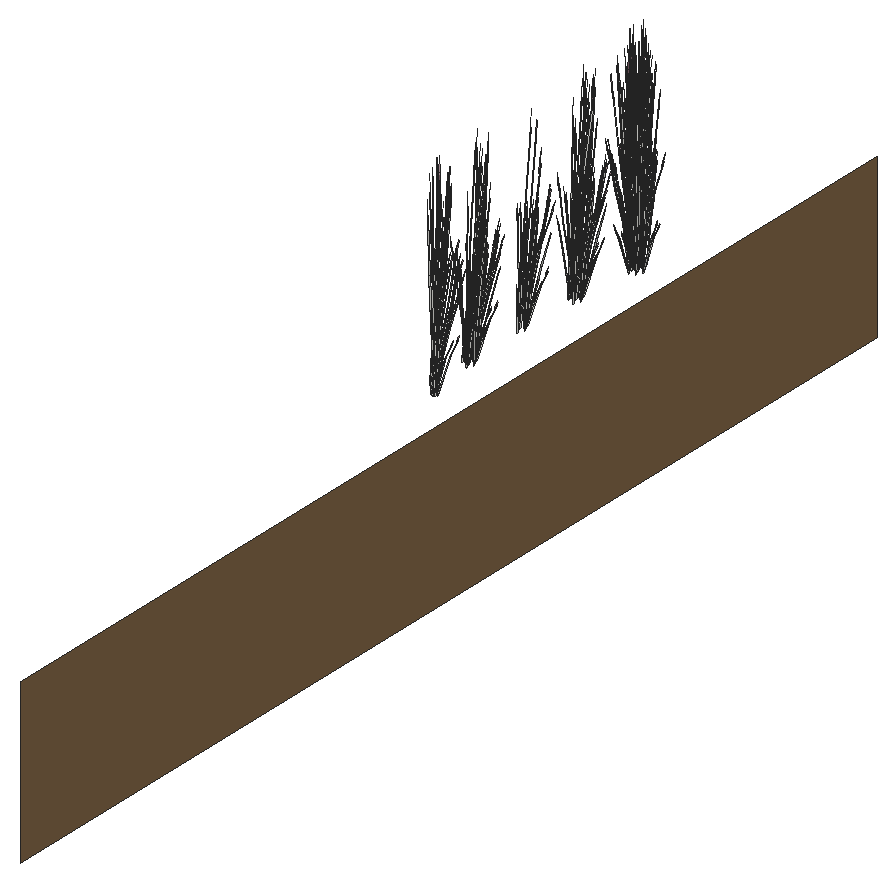
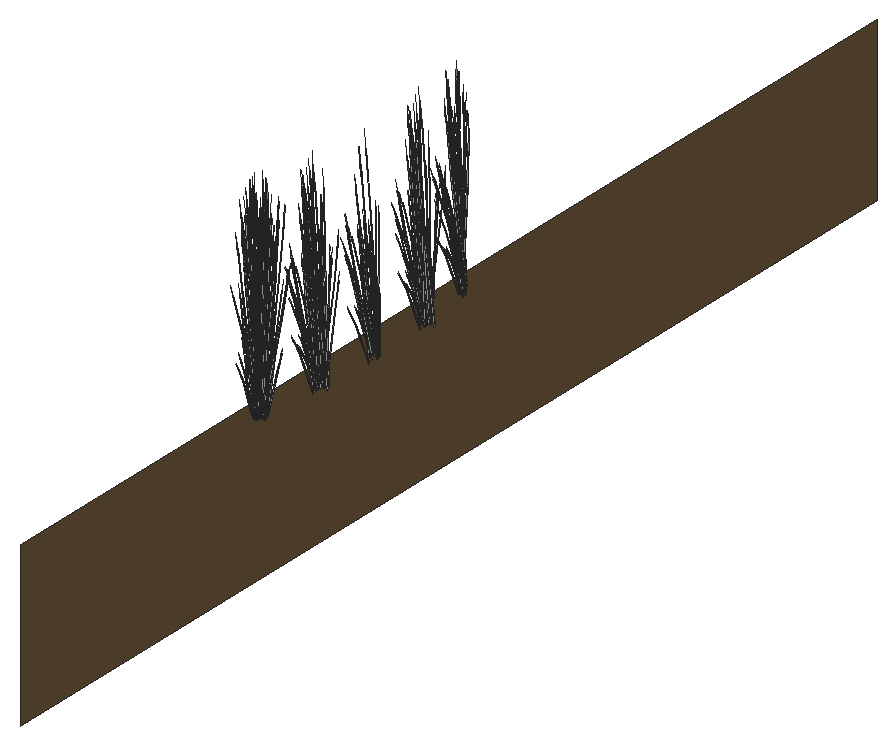
# SketchUp Ruby script. Lengths in inches.
U = 1.inch
M = Sketchup.active_model
def pt(a) = Geom::Point3d.new(a.map { |v| v * U })
def face(e, loops, mat)
  f = e.add_face(loops[0].map { |a| pt(a) })
  loops[1..].each { |l| e.add_face(l.map { |a| pt(a) }).erase! }
  f.material = f.back_material = mat if mat
  f
end
# faces: each face lists its corners as indices into pts; further lists are holes
def faces(e, pts, list, mat = nil) = list.each { |f| face(e, (f[0].is_a?(Array) ? f : [f]).map { |l| l.map { |i| pts[i] } }, mat) }
# xy, xz, yz: faces in a plane at the given z, y or x. An outline is a flat list of corners, or four numbers for a rectangle; further outlines are holes
def ring(l) = l.size == 4 ? [[l[0], l[1]], [l[2], l[1]], [l[2], l[3]], [l[0], l[3]]] : l.each_slice(2).to_a
def flat(e, list, mat, &to3) = list.each { |f| face(e, (f[0].is_a?(Array) ? f : [f]).map { |l| ring(l).map { |u, v| to3.(u, v) } }, mat) }
def xy(e, z, list, mat = nil) = flat(e, list, mat) { |x, y| [x, y, z] }
def xz(e, y, list, mat = nil) = flat(e, list, mat) { |x, z| [x, y, z] }
def yz(e, x, list, mat = nil) = flat(e, list, mat) { |y, z| [x, y, z] }
def lines(e, pts, list) = list.each { |a, b| e.add_line(pt(pts[a]), pt(pts[b])) }
# prism: a flat outline (further loops are holes) pulled along v
def prism(e, loops, v, mat = nil)
  f = face(e, loops, mat); d = Geom::Vector3d.new(v.map { |x| x * U })
  f.pushpull(f.normal.samedirection?(d) ? d.length : -d.length)
end
def box(e, o, s, mat = nil) = prism(e, [[o, [o[0] + s[0], o[1], o[2]], [o[0] + s[0], o[1] + s[1], o[2]], [o[0], o[1] + s[1], o[2]]]], [0, 0, s[2]], mat)
def at(x, y, z, deg = 0) = Geom::Transformation.translation(pt([x, y, z])) * Geom::Transformation.rotation(ORIGIN, Z_AXIS, deg.degrees)
def axes(o, x, y, z) = Geom::Transformation.new([*x, 0, *y, 0, *z, 0, *pt(o).to_a, 1])
def part(name) = M.definitions.add(name)
# library, detail: a bought-in or finely detailed component or shape, given as its bounding box
def library(name, o, s) = part(name).tap { |d| box(d.entities, o, s) }
def detail(e, o, s) = box(e.add_group.entities, o, s)
def put(e, d, t, mat = nil) = e.add_instance(d, t).tap { |i| i.material = mat if mat }
def group(e, t, mat = nil) = e.add_group.tap { |g| g.transformation = t; g.material = mat if mat }.entities
root = M.entities
M.materials.add("LightPink_Translucent").color = [144, 107, 117]
M.materials["LightPink_Translucent"].alpha = 0.75
M.materials.add("Soil_03_1K").color = [122, 96, 67]
c1 = part("blade")
p = [[2.15,0.21,22],[0,0.17,0],[0.09,0.45,0],[2.18,0.31,22],[2.29,0.31,22],[0.38,0.45,0],
  [2.48,0.24,33],[2.49,0.24,33],[2.48,0.22,33]]
faces(c1.entities,p,[[0,1,2,3],[4,5,2,3],[6,3,4,7],[8,0,3,6]])
c2 = part("seeds")
p = [[0.3,-0.1,1.38],[-0.01,-0.03,1.59],[-0.01,-0.03,0.03],[0.14,-0.07,-0.07],[0.29,-0.03,3],[0.15,0.01,3.11]]
faces(c2.entities,p,[[0,1,2,3],[1,0,4,5]],"LightPink_Translucent")
c3 = part("blade with seeds")
put(c3.entities,c1,at(0,0,0))
put(c3.entities,c2,axes([2.4,0.25,30.99],[1.5799,-0.05474,1.17369],[-0.12525,1.92788,0.29478],[-0.07173,-0.02425,1.56792]))
yz(root,410.57,[[0,-48,316.3,0]],"Soil_03_1K")
put(root,c3,axes([402.34,162.62,2.29],[0.15345,0.53576,-0.06012],[-0.43845,0.18773,0],[0.00536,0.01871,1.72173]))
put(root,c3,axes([402.51,163.2,2.03],[-0.32928,-0.11539,-0.30978],[0.08291,-0.40636,0.30978],[-0.06638,0.04686,1.38974]))
put(root,c3,axes([403.78,161.65,2.375],[0.44133,0,0],[0,0.52122,-0.51607],[0,0.11871,1.63711]))
put(root,c3,axes([403.61,161.92,2.2],[-0.44111,-0.00373,-0.04976],[0,-0.52122,0.49943],[-0.01386,0.11865,1.58352]))
put(root,c3,axes([402.65,161.47,2.67],[0.39748,0.22252,-0.29095],[-0.19139,0.46966,-0.50002],[0.01249,0.11531,1.59708]))
put(root,c3,axes([403.42,162.81,4.53],[0.20082,0.29199,-0.35414],[-0.2293,0.2764,0.4572],[0.1165,0.04206,0.87481]))
put(root,c3,axes([403.52,162,2.03],[-0.24637,0.29097,-0.30978],[-0.24637,-0.29097,0.30978],[0,0.09372,1.38974]))
put(root,c3,axes([402.46,162.02,2.67],[0.04113,0.53214,-0.29095],[-0.42835,0.03218,-0.50002],[-0.07543,0.07088,1.59708]))
put(root,c3,axes([402.61,161.82,2.21],[-0.17124,0.42022,-0.44739],[-0.35581,-0.20224,0.21531],[0,0.09687,1.43643]))
put(root,c3,axes([402.62,163.02,2.33],[0.44186,0.15158,0.30756],[-0.11054,0.54181,-0.36492],[-0.07313,0.06781,1.64885]))
put(root,c3,axes([402.59,163.39,2.02],[-0.33032,0.23318,-0.49651],[-0.19744,-0.41812,0],[-0.07523,0.05311,1.57504]))
put(root,c3,axes([403.6875,162.01,2.02],[0,0.46636,-0.49651],[-0.39487,0,0],[0,0.10622,1.57504]))
put(root,c3,axes([402.7,162.06,3.875],[-0.1311,-0.08035,1.71376],[0.27131,-0.33708,0.13857],[0.16909,0.15206,0.73262]))
put(root,c3,axes([403.18,162.97,2.77],[-0.19872,-0.13409,1.1486],[0.2566,-0.13625,0.84392],[0.06921,0.11541,0.25299]))
put(root,c3,axes([402.89,163.3125,2.375],[0.22066,0.46731,0],[-0.36918,0.26061,-0.51607],[-0.08408,0.05936,1.63711]))
put(root,c3,axes([403.24,163.47,1.49],[0.02571,-0.06733,1.76342],[0.32373,-0.19829,-0.26939],[0.09815,0.10263,0.30037]))
put(root,c3,axes([402.7,161.46,2.84],[-0.00964,-0.43909,1.41272],[0.43635,0.11382,0.59816],[-0.1032,0.24027,1.3335]))
put(root,c3,axes([402.8125,161.94,2.09],[0.12941,0.42699,-0.69212],[-0.37279,0.15378,-0.18165],[0.0143,0.14459,1.52773]))
put(root,c3,axes([402.74,163.16,4.68],[0.34827,-0.11086,-0.51099],[0.06092,0.41983,-0.3958],[0.09354,0.12031,0.97773]))
put(root,c3,axes([403.22,163.58,2.67],[-0.22633,-0.01463,1.0506],[0.14947,-0.31064,0.58006],[0.08941,0.11036,0.8241]))
put(root,c3,axes([402.48,162.83,2.59],[0.00623,-0.15459,1.43002],[0.29764,-0.17268,-0.30754],[0.09188,0.18503,0.61141]))
put(root,c3,axes([401.73,163.46,1.49],[0.05712,-0.02538,1.76342],[0.34359,0.13968,-0.26939],[0.01005,0.15742,0.30037]))
put(root,c3,axes([401.21,163.05,5],[0.25266,0.31335,-0.5672],[-0.2669,0.27442,-0.43934],[-0.03844,0.15921,1.08528]))
put(root,c3,axes([400.9375,163.52,2.82],[0.32063,-0.08258,0.06507],[0.07371,0.33271,-0.86304],[-0.02033,0.16842,0.7736]))
put(root,c3,axes([401.96,163.35,4.68],[0.34695,0.11691,-0.51099],[-0.11892,0.40083,-0.3958],[0.03181,0.16138,0.97773]))
put(root,c3,axes([402.16,162.53,3.875],[-0.08068,-0.14973,1.71376],[0.3728,-0.12606,0.13857],[0.08426,0.23506,0.73262]))
put(root,c3,axes([401.8,163.6,4.53],[-0.1064,0.35863,-0.35414],[-0.31043,-0.1046,0.4572],[0.02846,0.14439,0.87481]))
put(root,c3,axes([401.5,162.6,3.875],[-0.00864,-0.17899,1.71376],[0.37441,0.11874,0.13857],[-0.02316,0.25508,0.73262]))
put(root,c3,axes([401.84,163.28,4.98],[0.16845,0.3792,-0.71045],[-0.34676,0.21133,0.08574],[0.03939,0.18322,1.00501]))
put(root,c3,axes([399.77,178.33,4.98],[0.00918,-0.43138,-0.71045],[0.38672,0.02897,0.08574],[0.04081,-0.18275,1.00501]))
put(root,c3,axes([399.34,178.12,3.875],[-0.06572,0.16029,1.71376],[-0.27569,-0.33172,0.13857],[0.12437,-0.20675,0.73262]))
put(root,c3,axes([399.93,178.08,4.53],[0.23881,-0.24554,-0.35414],[0.22606,0.28036,0.4572],[0.0344,-0.14245,0.87481]))
put(root,c3,axes([400.23,177.93,1.49],[-0.05283,-0.03674,1.76342],[-0.13569,-0.41045,-0.26939],[0.09154,-0.11138,0.30037]))
put(root,c3,axes([400.23,179.08,4.98],[0.18436,-0.36797,-0.71045],[0.32306,0.26151,0.08574],[0.11008,-0.13332,1.00501]))
put(root,c3,axes([400.22,178.91,4.68],[-0.09067,-0.42583,-0.51099],[0.34336,-0.07449,-0.3958],[0.0984,-0.11438,0.97773]))
put(root,c3,axes([400.49,178.75,2.59],[-0.12609,-0.01381,1.43002],[-0.12917,-0.37055,-0.30754],[0.1549,-0.10482,0.61141]))
put(root,c3,axes([398.93,178.9,2.06],[0.23773,-0.35053,-0.62353],[0.29532,0.31785,-0.16365],[0.09526,-0.08744,1.37633]))
put(root,c3,axes([400.64,178.07,2.77],[-0.11756,0.2374,1.1486],[-0.10105,-0.31895,0.84392],[0.09709,-0.07992,0.25299]))
put(root,c3,axes([400.47,178.96,4.53],[0.30722,-0.06665,-0.35414],[0.08112,0.381,0.4572],[0.08804,-0.10234,0.87481]))
put(root,c3,axes([400.38,179.86,4.68],[0.09562,-0.42421,-0.51099],[0.32782,0.1454,-0.3958],[0.13199,-0.0389,0.97773]))
put(root,c3,axes([399.86,178.13,2.375],[0.22066,-0.46731,0],[0.36918,0.26061,-0.51607],[0.08408,0.05936,1.63711]))
put(root,c3,axes([400.73,179.98,1.98],[-0.22732,0.05597,1.41583],[-0.03618,-0.44548,0.08104],[0.15921,-0.06743,0.80566]))
put(root,c3,axes([401.14,179.58,2.26],[-0.21881,-0.29821,-0.06488],[0.23965,-0.27324,-0.29416],[0.0679,-0.01924,0.97024]))
put(root,c3,axes([399.67,178.375,2.48],[-0.33032,-0.23318,0.49651],[0.19744,-0.41812,0],[0.07523,0.05311,1.57504]))
put(root,c3,axes([400.32,180.01,4.98],[0.31014,-0.20596,-0.71045],[0.17284,0.42397,0.08574],[0.14985,-0.04816,1.00501]))
put(root,c3,axes([398.26,178.96,1.59],[-0.3474,0.18671,1.28929],[-0.11057,-0.53572,0.50096],[0.21332,0.00891,1.46642]))
put(root,c3,axes([400.98,179.6875,1.49],[-0.01845,-0.0708,1.76342],[0.12793,-0.41416,-0.26939],[0.12905,-0.00596,0.30037]))
put(root,c3,axes([399.16,179.24,2.67],[0.35635,-0.30962,-0.29095],[0.23697,0.43749,-0.50002],[0.08792,0.04443,1.59708]))
put(root,c3,axes([400.58,180.05,4.53],[0.29332,0.1301,-0.35414],[-0.08555,0.37955,0.4572],[0.11809,-0.0348,0.87481]))
put(root,c3,axes([400.06,178.41,2.02],[0.33032,0.23318,-0.49651],[-0.19744,0.41812,0],[0.07523,0.05311,1.57504]))
put(root,c3,axes([399.78,179.58,3.875],[-0.14639,0.01056,1.71376],[0.09712,-0.45778,0.13857],[0.20862,0.02831,0.73262]))
put(root,c3,axes([399.97,178.59,2.03],[0.08291,0.40636,-0.30978],[-0.32928,0.11539,0.30978],[0.06638,0.04686,1.38974]))
put(root,c3,axes([399.38,180.81,2.18],[0.37054,-0.15823,-0.19198],[0.1302,0.45581,0.00008],[0.0409,-0.01749,1.73897]))
put(root,c3,axes([399.58,179.31,2.06],[0.36714,0.07646,-0.62353],[-0.07747,0.47163,-0.16365],[0.10956,0.05715,1.37633]))
put(root,c3,axes([401.2,180.13,2.77],[-0.21807,0.07699,1.1486],[0.10265,-0.31819,0.84392],[0.11568,0.02177,0.25299]))
put(root,c3,axes([399.39,179.46,2.21],[0.21202,0.39143,-0.44739],[-0.32115,0.27564,0.21531],[0.06861,0.04843,1.43643]))
put(root,c3,axes([400.82,181.11,3.93],[-0.06755,-0.39203,-0.03492],[0.31928,-0.09013,-0.15832],[0.06667,0.02485,0.52218]))
put(root,c3,axes([400.79,180.64,2.59],[-0.085,-0.1147,1.43002],[0.1106,-0.37943,-0.30754],[0.17198,0.0514,0.61141]))
put(root,c3,axes([400.01,180.87,4.98],[0.35281,0.01123,-0.71045],[-0.0237,0.47284,0.08574],[0.14947,0.0499,1.00501]))
put(root,c3,axes([400.59,179.91,2.375],[0.44133,0,0],[0,0.52122,-0.51607],[0,0.11871,1.63711]))
put(root,c3,axes([400.22,181.07,4.53],[0.20082,0.29199,-0.35414],[-0.2293,0.2764,0.4572],[0.1165,0.04206,0.87481]))
put(root,c3,axes([399.5,180.32,3.875],[-0.1311,-0.08035,1.71376],[0.27131,-0.33708,0.13857],[0.16909,0.15206,0.73262]))
put(root,c3,axes([399.99,181.23,2.77],[-0.19872,-0.13409,1.1486],[0.2566,-0.13625,0.84392],[0.06921,0.11541,0.25299]))
put(root,c3,axes([400.04,181.73,1.49],[0.02571,-0.06733,1.76342],[0.32373,-0.19829,-0.26939],[0.09815,0.10263,0.30037]))
put(root,c3,axes([399.54,181.42,4.68],[0.34827,-0.11086,-0.51099],[0.06092,0.41983,-0.3958],[0.09354,0.12031,0.97773]))
put(root,c3,axes([400.02,181.84,2.67],[-0.22633,-0.01463,1.0506],[0.14947,-0.31064,0.58006],[0.08941,0.11036,0.8241]))
put(root,c3,axes([399.28,181.09,2.59],[0.00623,-0.15459,1.43002],[0.29764,-0.17268,-0.30754],[0.09188,0.18503,0.61141]))
put(root,c3,axes([399.21,197.96,1.49],[-0.05283,-0.03674,1.76342],[-0.13569,-0.41045,-0.26939],[0.09154,-0.11138,0.30037]))
put(root,c3,axes([399.21,199.12,4.98],[0.18436,-0.36797,-0.71045],[0.32306,0.26151,0.08574],[0.11008,-0.13332,1.00501]))
put(root,c3,axes([399.2,198.95,4.68],[-0.09067,-0.42583,-0.51099],[0.34336,-0.07449,-0.3958],[0.0984,-0.11438,0.97773]))
put(root,c3,axes([399.48,198.78,2.59],[-0.12609,-0.01381,1.43002],[-0.12917,-0.37055,-0.30754],[0.1549,-0.10482,0.61141]))
put(root,c3,axes([399.625,198.1,2.77],[-0.11756,0.2374,1.1486],[-0.10105,-0.31895,0.84392],[0.09709,-0.07992,0.25299]))
put(root,c3,axes([399.46,198.99,4.53],[0.30722,-0.06665,-0.35414],[0.08112,0.381,0.4572],[0.08804,-0.10234,0.87481]))
put(root,c3,axes([399.36,199.89,4.68],[0.09562,-0.42421,-0.51099],[0.32782,0.1454,-0.3958],[0.13199,-0.0389,0.97773]))
put(root,c3,axes([398.84,198.17,2.375],[0.22066,-0.46731,0],[0.36918,0.26061,-0.51607],[0.08408,0.05936,1.63711]))
put(root,c3,axes([399.71,200.01,1.98],[-0.22732,0.05597,1.41583],[-0.03618,-0.44548,0.08104],[0.15921,-0.06743,0.80566]))
put(root,c3,axes([400.125,199.62,2.26],[-0.21881,-0.29821,-0.06488],[0.23965,-0.27324,-0.29416],[0.0679,-0.01924,0.97024]))
put(root,c3,axes([399.3,200.05,4.98],[0.31014,-0.20596,-0.71045],[0.17284,0.42397,0.08574],[0.14985,-0.04816,1.00501]))
put(root,c3,axes([399.96,199.72,1.49],[-0.01845,-0.0708,1.76342],[0.12793,-0.41416,-0.26939],[0.12905,-0.00596,0.30037]))
put(root,c3,axes([399.5625,200.09,4.53],[0.29332,0.1301,-0.35414],[-0.08555,0.37955,0.4572],[0.11809,-0.0348,0.87481]))
put(root,c3,axes([399.04,198.45,2.02],[0.33032,0.23318,-0.49651],[-0.19744,0.41812,0],[0.07523,0.05311,1.57504]))
put(root,c3,axes([398.76,199.62,3.875],[-0.14639,0.01056,1.71376],[0.09712,-0.45778,0.13857],[0.20862,0.02831,0.73262]))
put(root,c3,axes([398.5625,199.34,2.06],[0.36714,0.07646,-0.62353],[-0.07747,0.47163,-0.16365],[0.10956,0.05715,1.37633]))
put(root,c3,axes([400.19,200.17,2.77],[-0.21807,0.07699,1.1486],[0.10265,-0.31819,0.84392],[0.11568,0.02177,0.25299]))
put(root,c3,axes([399.81,201.15,3.93],[-0.06755,-0.39203,-0.03492],[0.31928,-0.09013,-0.15832],[0.06667,0.02485,0.52218]))
put(root,c3,axes([399.78,200.68,2.59],[-0.085,-0.1147,1.43002],[0.1106,-0.37943,-0.30754],[0.17198,0.0514,0.61141]))
put(root,c3,axes([399,200.91,4.98],[0.35281,0.01123,-0.71045],[-0.0237,0.47284,0.08574],[0.14947,0.0499,1.00501]))
put(root,c3,axes([399.21,201.1,4.53],[0.20082,0.29199,-0.35414],[-0.2293,0.2764,0.4572],[0.1165,0.04206,0.87481]))
put(root,c3,axes([398.49,200.35,3.875],[-0.1311,-0.08035,1.71376],[0.27131,-0.33708,0.13857],[0.16909,0.15206,0.73262]))
put(root,c3,axes([399.03,201.77,1.49],[0.02571,-0.06733,1.76342],[0.32373,-0.19829,-0.26939],[0.09815,0.10263,0.30037]))
put(root,c3,axes([398.52,201.45,4.68],[0.34827,-0.11086,-0.51099],[0.06092,0.41983,-0.3958],[0.09354,0.12031,0.97773]))
put(root,c3,axes([399.99,216.5,2.59],[-0.10032,0.0944,1.43002],[-0.30046,-0.16522,-0.30754],[0.05569,-0.20547,0.61141]))
put(root,c3,axes([400.24,217.2,4.98],[0.00918,-0.43138,-0.71045],[0.38672,0.02897,0.08574],[0.04081,-0.18275,1.00501]))
put(root,c3,axes([399.8,216.98,3.875],[-0.06572,0.16029,1.71376],[-0.27569,-0.33172,0.13857],[0.12437,-0.20675,0.73262]))
put(root,c3,axes([400.4,216.94,4.53],[0.23881,-0.24554,-0.35414],[0.22606,0.28036,0.4572],[0.0344,-0.14245,0.87481]))
put(root,c3,axes([400.69,216.79,1.49],[-0.05283,-0.03674,1.76342],[-0.13569,-0.41045,-0.26939],[0.09154,-0.11138,0.30037]))
put(root,c3,axes([400.69,217.95,4.98],[0.18436,-0.36797,-0.71045],[0.32306,0.26151,0.08574],[0.11008,-0.13332,1.00501]))
put(root,c3,axes([400.68,217.78,4.68],[-0.09067,-0.42583,-0.51099],[0.34336,-0.07449,-0.3958],[0.0984,-0.11438,0.97773]))
put(root,c3,axes([399,216.81,2.02],[0.33032,-0.23318,-0.49651],[0.19744,0.41812,0],[0.07523,-0.05311,1.57504]))
put(root,c3,axes([400.96,217.61,2.59],[-0.12609,-0.01381,1.43002],[-0.12917,-0.37055,-0.30754],[0.1549,-0.10482,0.61141]))
put(root,c3,axes([399.39,217.76,2.06],[0.23773,-0.35053,-0.62353],[0.29532,0.31785,-0.16365],[0.09526,-0.08744,1.37633]))
put(root,c3,axes([401.1,216.93,2.77],[-0.11756,0.2374,1.1486],[-0.10105,-0.31895,0.84392],[0.09709,-0.07992,0.25299]))
put(root,c3,axes([400.9375,217.82,4.53],[0.30722,-0.06665,-0.35414],[0.08112,0.381,0.4572],[0.08804,-0.10234,0.87481]))
put(root,c3,axes([399.08,216.99,2.03],[0.32928,0.11539,-0.30978],[-0.08291,0.40636,0.30978],[0.06638,-0.04686,1.38974]))
put(root,c3,axes([400.84,218.72,4.68],[0.09562,-0.42421,-0.51099],[0.32782,0.1454,-0.3958],[0.13199,-0.0389,0.97773]))
put(root,c3,axes([400.32,217,2.375],[0.22066,-0.46731,0],[0.36918,0.26061,-0.51607],[0.08408,0.05936,1.63711]))
put(root,c3,axes([401.19,218.84,1.98],[-0.22732,0.05597,1.41583],[-0.03618,-0.44548,0.08104],[0.15921,-0.06743,0.80566]))
put(root,c3,axes([401.61,218.45,2.26],[-0.21881,-0.29821,-0.06488],[0.23965,-0.27324,-0.29416],[0.0679,-0.01924,0.97024]))
put(root,c3,axes([400.13,217.24,2.48],[-0.33032,-0.23318,0.49651],[0.19744,-0.41812,0],[0.07523,0.05311,1.57504]))
put(root,c3,axes([400.78,218.88,4.98],[0.31014,-0.20596,-0.71045],[0.17284,0.42397,0.08574],[0.14985,-0.04816,1.00501]))
put(root,c3,axes([398.73,217.83,1.59],[-0.3474,0.18671,1.28929],[-0.11057,-0.53572,0.50096],[0.21332,0.00891,1.46642]))
put(root,c3,axes([399.66,217.97,2.62],[0.06809,-0.4162,0.1448],[0.33266,0.07225,-0.41347],[0.06054,0.04274,1.26744]))
put(root,c3,axes([401.44,218.55,1.49],[-0.01845,-0.0708,1.76342],[0.12793,-0.41416,-0.26939],[0.12905,-0.00596,0.30037]))
put(root,c3,axes([399.625,218.1,2.67],[0.35635,-0.30962,-0.29095],[0.23697,0.43749,-0.50002],[0.08792,0.04443,1.59708]))
put(root,c3,axes([401.04,218.92,4.53],[0.29332,0.1301,-0.35414],[-0.08555,0.37955,0.4572],[0.11809,-0.0348,0.87481]))
put(root,c3,axes([400.53,217.28,2.02],[0.33032,0.23318,-0.49651],[-0.19744,0.41812,0],[0.07523,0.05311,1.57504]))
put(root,c3,axes([400.24,218.45,3.875],[-0.14639,0.01056,1.71376],[0.09712,-0.45778,0.13857],[0.20862,0.02831,0.73262]))
put(root,c3,axes([400.43,217.45,2.03],[0.08291,0.40636,-0.30978],[-0.32928,0.11539,0.30978],[0.06638,0.04686,1.38974]))
put(root,c3,axes([399.85,219.68,2.18],[0.37054,-0.15823,-0.19198],[0.1302,0.45581,0.00008],[0.0409,-0.01749,1.73897]))
put(root,c3,axes([400.04,218.17,2.06],[0.36714,0.07646,-0.62353],[-0.07747,0.47163,-0.16365],[0.10956,0.05715,1.37633]))
put(root,c3,axes([401.67,218.99,2.77],[-0.21807,0.07699,1.1486],[0.10265,-0.31819,0.84392],[0.11568,0.02177,0.25299]))
put(root,c3,axes([399.85,218.32,2.21],[0.21202,0.39143,-0.44739],[-0.32115,0.27564,0.21531],[0.06861,0.04843,1.43643]))
put(root,c3,axes([401.29,219.98,3.93],[-0.06755,-0.39203,-0.03492],[0.31928,-0.09013,-0.15832],[0.06667,0.02485,0.52218]))
put(root,c3,axes([400.79,218.7,2.48],[0,-0.46636,0.49651],[0.39487,0,0],[0,0.10622,1.57504]))
put(root,c3,axes([401.26,219.51,2.59],[-0.085,-0.1147,1.43002],[0.1106,-0.37943,-0.30754],[0.17198,0.0514,0.61141]))
put(root,c3,axes([400.48,219.74,4.98],[0.35281,0.01123,-0.71045],[-0.0237,0.47284,0.08574],[0.14947,0.0499,1.00501]))
put(root,c3,axes([401.05,218.78,2.375],[0.44133,0,0],[0,0.52122,-0.51607],[0,0.11871,1.63711]))
put(root,c3,axes([399.92,218.59,2.67],[0.39748,0.22252,-0.29095],[-0.19139,0.46966,-0.50002],[0.01249,0.11531,1.59708]))
put(root,c3,axes([400.6875,219.93,4.53],[0.20082,0.29199,-0.35414],[-0.2293,0.2764,0.4572],[0.1165,0.04206,0.87481]))
put(root,c3,axes([400.95,219.13,2.02],[0,0.46636,-0.49651],[-0.39487,0,0],[0,0.10622,1.57504]))
put(root,c3,axes([399.97,219.18,3.875],[-0.1311,-0.08035,1.71376],[0.27131,-0.33708,0.13857],[0.16909,0.15206,0.73262]))
put(root,c3,axes([400.45,220.1,2.77],[-0.19872,-0.13409,1.1486],[0.2566,-0.13625,0.84392],[0.06921,0.11541,0.25299]))
put(root,c3,axes([400.51,220.6,1.49],[0.02571,-0.06733,1.76342],[0.32373,-0.19829,-0.26939],[0.09815,0.10263,0.30037]))
put(root,c3,axes([400,220.28,4.68],[0.34827,-0.11086,-0.51099],[0.06092,0.41983,-0.3958],[0.09354,0.12031,0.97773]))
put(root,c3,axes([400.48,220.71,2.67],[-0.22633,-0.01463,1.0506],[0.14947,-0.31064,0.58006],[0.08941,0.11036,0.8241]))
put(root,c3,axes([399.75,219.95,2.59],[0.00623,-0.15459,1.43002],[0.29764,-0.17268,-0.30754],[0.09188,0.18503,0.61141]))
put(root,c3,axes([399.43,219.65,3.875],[-0.08068,-0.14973,1.71376],[0.3728,-0.12606,0.13857],[0.08426,0.23506,0.73262]))
put(root,c3,axes([402.72,236.22,2.59],[-0.10032,0.0944,1.43002],[-0.30046,-0.16522,-0.30754],[0.05569,-0.20547,0.61141]))
put(root,c3,axes([402.27,236.55,4.98],[-0.16845,-0.3792,-0.71045],[0.34676,-0.21133,0.08574],[-0.03939,-0.18322,1.00501]))
put(root,c3,axes([401.98,235.7,1.49],[-0.0592,0.0168,1.76342],[-0.32738,-0.18913,-0.26939],[0.00549,-0.15776,0.30037]))
put(root,c3,axes([402.97,236.92,4.98],[0.00918,-0.43138,-0.71045],[0.38672,0.02897,0.08574],[0.04081,-0.18275,1.00501]))
put(root,c3,axes([402.3,236.22,4.53],[0.1064,-0.35863,-0.35414],[0.31043,0.1046,0.4572],[-0.02846,-0.14439,0.87481]))
put(root,c3,axes([402.53,236.7,3.875],[-0.06572,0.16029,1.71376],[-0.27569,-0.33172,0.13857],[0.12437,-0.20675,0.73262]))
put(root,c3,axes([402.14,236.47,4.68],[-0.34695,-0.11691,-0.51099],[0.11892,-0.40083,-0.3958],[-0.03181,-0.16138,0.97773]))
put(root,c3,axes([402.35,235.47,2.77],[0.04528,0.27194,1.1486],[-0.25117,-0.15062,0.84392],[0.02703,-0.13924,0.25299]))
put(root,c3,axes([402.89,236.77,4.68],[-0.25266,-0.31335,-0.51099],[0.2669,-0.27442,-0.3958],[0.03844,-0.15921,0.97773]))
put(root,c3,axes([403.13,236.66,4.53],[0.23881,-0.24554,-0.35414],[0.22606,0.28036,0.4572],[0.0344,-0.14245,0.87481]))
put(root,c3,axes([401.49,237.97,2.1],[-0.14494,-0.47823,-0.69835],[0.41752,-0.17223,-0.18329],[-0.01602,-0.16194,1.54149]))
put(root,c3,axes([403.43,236.51,1.49],[-0.05283,-0.03674,1.76342],[-0.13569,-0.41045,-0.26939],[0.09154,-0.11138,0.30037]))
put(root,c3,axes([403.42,237.67,4.98],[0.18436,-0.36797,-0.71045],[0.32306,0.26151,0.08574],[0.11008,-0.13332,1.00501]))
put(root,c3,axes([401.43,236.6,2.375],[-0.22066,-0.46731,0],[0.36918,-0.26061,-0.51607],[0.08408,-0.05936,1.63711]))
put(root,c3,axes([403.41,237.49,4.68],[-0.09067,-0.42583,-0.51099],[0.34336,-0.07449,-0.3958],[0.0984,-0.11438,0.97773]))
put(root,c3,axes([401.92,236.03,2.13],[-0.2439,0.26754,-0.03893],[-0.22348,-0.29302,-0.17649],[-0.01573,-0.08303,0.58215]))
put(root,c3,axes([400.63,237.9,2.02],[0,-0.46636,-0.49651],[0.39487,0,0],[0,-0.10622,1.57504]))
put(root,c3,axes([401.73,236.52,2.02],[0.33032,-0.23318,-0.49651],[0.19744,0.41812,0],[0.07523,-0.05311,1.57504]))
put(root,c3,axes([403.69,237.33,2.59],[-0.12609,-0.01381,1.43002],[-0.12917,-0.37055,-0.30754],[0.1549,-0.10482,0.61141]))
put(root,c3,axes([402.12,237.48,2.06],[0.23773,-0.35053,-0.62353],[0.29532,0.31785,-0.16365],[0.09526,-0.08744,1.37633]))
put(root,c3,axes([403.84,236.65,2.77],[-0.11756,0.2374,1.1486],[-0.10105,-0.31895,0.84392],[0.09709,-0.07992,0.25299]))
put(root,c3,axes([403.67,237.54,4.53],[0.30722,-0.06665,-0.35414],[0.08112,0.381,0.4572],[0.08804,-0.10234,0.87481]))
put(root,c3,axes([401.71,238.09,2.21],[0.17124,-0.42022,-0.44739],[0.35581,0.20224,0.21531],[0,-0.09687,1.43643]))
put(root,c3,axes([401.86,237.89,2.67],[-0.04113,-0.53214,-0.29095],[0.42835,-0.03218,-0.50002],[0.07543,-0.07088,1.59708]))
put(root,c3,axes([400.8,237.91,2.03],[0.24637,-0.29097,-0.30978],[0.24637,0.29097,0.30978],[0,-0.09372,1.38974]))
put(root,c3,axes([401.67,238.44,2.67],[-0.39748,-0.22252,-0.29095],[0.19139,-0.46966,-0.50002],[-0.01249,-0.11531,1.59708]))
put(root,c3,axes([401.81,236.71,2.03],[0.32928,0.11539,-0.30978],[-0.08291,0.40636,0.30978],[0.06638,-0.04686,1.38974]))
put(root,c3,axes([401.92,238.3,2.43],[0.39767,0.22603,0.24065],[-0.19139,0.46966,0.50002],[0,-0.10827,1.60543]))
put(root,c3,axes([401.77,238.9375,2.4375],[0.09355,-0.55261,-0.23429],[0.44354,0.09633,0.51271],[-0.0775,-0.07631,1.5644]))
put(root,c3,axes([401.79,237.99,2.72],[-0.38326,0.02879,0.44739],[-0.03466,-0.47788,-0.21531],[0.06861,-0.04843,1.43643]))
put(root,c3,axes([400.8,238.34,2.48],[0,0.46636,0.49651],[-0.39487,0,0],[0,-0.10622,1.57504]))
put(root,c3,axes([403.57,238.44,4.68],[0.09562,-0.42421,-0.51099],[0.32782,0.1454,-0.3958],[0.13199,-0.0389,0.97773]))
put(root,c3,axes([403.06,236.71,2.375],[0.22066,-0.46731,0],[0.36918,0.26061,-0.51607],[0.08408,0.05936,1.63711]))
put(root,c3,axes([401.78,238.16,2.36],[0.15345,0.52148,0.45755],[-0.43845,0.18134,0.17955],[0.00536,-0.09582,1.58856]))
put(root,c3,axes([403.92,238.56,1.98],[-0.22732,0.05597,1.41583],[-0.03618,-0.44548,0.08104],[0.15921,-0.06743,0.80566]))
put(root,c3,axes([404.34,238.17,2.26],[-0.21881,-0.29821,-0.06488],[0.23965,-0.27324,-0.29416],[0.0679,-0.01924,0.97024]))
put(root,c3,axes([401.7,238.57,2.72],[-0.17124,0.42022,0.44739],[-0.35581,-0.20224,-0.21531],[0,-0.09687,1.43643]))
put(root,c3,axes([402.33,238.2,2.21],[0,-0.53961,0],[0.44133,0,0],[0,0,1.79456]))
put(root,c3,axes([402.87,236.96,2.48],[-0.33032,-0.23318,0.49651],[0.19744,-0.41812,0],[0.07523,0.05311,1.57504]))
put(root,c3,axes([403.51,238.59,4.98],[0.31014,-0.20596,-0.71045],[0.17284,0.42397,0.08574],[0.14985,-0.04816,1.00501]))
put(root,c3,axes([402.12,237.86,2.36],[-0.29264,0.42323,0.45755],[-0.34767,-0.3736,0.17955],[0.07055,-0.04224,1.58856]))
put(root,c3,axes([402.44,238.62,2.3],[-0.32829,-0.4014,-0.06131],[0.32849,-0.40164,0],[-0.01146,-0.01402,1.75571]))
put(root,c3,axes([401.61,237.17,2.47],[-0.10196,0.46348,0.17642],[-0.3731,-0.13116,0.35086],[0.06445,-0.00226,1.60407]))
put(root,c3,axes([401.46,237.54,1.59],[-0.3474,0.18671,1.28929],[-0.11057,-0.53572,0.50096],[0.21332,0.00891,1.46642]))
put(root,c3,axes([402.39,237.68,2.62],[0.06809,-0.4162,0.1448],[0.33266,0.07225,-0.41347],[0.06054,0.04274,1.26744]))
put(root,c3,axes([401.82,238.67,2.36],[0.44609,0.09826,0.45755],[-0.09078,0.55493,0.17955],[-0.06519,-0.05359,1.58856]))
put(root,c3,axes([404.17,238.27,1.49],[-0.01845,-0.0708,1.76342],[0.12793,-0.41416,-0.26939],[0.12905,-0.00596,0.30037]))
put(root,c3,axes([402.25,237.79,2.72],[-0.21202,-0.39143,0.44739],[0.32115,-0.27564,-0.21531],[0.06861,0.04843,1.43643]))
put(root,c3,axes([401.58,239.56,2.47],[0.37926,-0.12378,0.17642],[0.09365,0.46065,0.35086],[-0.03382,-0.06712,1.60407]))
put(root,c3,axes([402.36,237.82,2.67],[0.35635,-0.30962,-0.29095],[0.23697,0.43749,-0.50002],[0.08792,0.04443,1.59708]))
put(root,c3,axes([403.78,238.63,4.53],[0.29332,0.1301,-0.35414],[-0.08555,0.37955,0.4572],[0.11809,-0.0348,0.87481]))
put(root,c3,axes([403.26,236.99,2.02],[0.33032,0.23318,-0.49651],[-0.19744,0.41812,0],[0.07523,0.05311,1.57504]))
put(root,c3,axes([402.63,238.32,2.21],[0.39487,0,0],[0,0.48281,0],[0,0,1.78407]))
put(root,c3,axes([402.74,237.19,2.47],[-0.37926,0.12378,0.17642],[-0.09365,-0.46065,0.35086],[0.03382,0.06712,1.60407]))
put(root,c3,axes([402.98,238.16,3.875],[-0.14639,0.01056,1.71376],[0.09712,-0.45778,0.13857],[0.20862,0.02831,0.73262]))
put(root,c3,axes([403.17,237.17,2.03],[0.08291,0.40636,-0.30978],[-0.32928,0.11539,0.30978],[0.06638,0.04686,1.38974]))
put(root,c3,axes([402.5,238.08,2.38],[-0.44609,-0.09826,0.49198],[0.09078,-0.55493,0.19306],[0.06519,0.05359,1.70813]))
put(root,c3,axes([402.15,239.45,2.2],[-0.11516,-0.40207,0],[0.32884,-0.1408,0],[0,0,1.54371]))
put(root,c3,axes([401.93,239.07,2.62],[-0.06809,0.4162,0.1448],[-0.33266,-0.07225,-0.41347],[-0.06054,-0.04274,1.26744]))
put(root,c3,axes([402.58,239.39,2.18],[0.37054,-0.15823,-0.19198],[0.1302,0.45581,0.00008],[0.0409,-0.01749,1.73897]))
put(root,c3,axes([402.71,239.58,2.47],[0.10196,-0.46348,0.17642],[0.3731,0.13116,0.35086],[-0.06445,0.00226,1.60407]))
put(root,c3,axes([402.62,238.53,2.21],[0.24637,0.30123,0],[-0.24637,0.30123,0],[0,0,1.69266]))
put(root,c3,axes([403.29,238.4,2.47],[-0.2773,-0.3397,0.17642],[0.27945,-0.32949,0.35086],[-0.03063,0.06937,1.60407]))
put(root,c3,axes([402.78,237.89,2.06],[0.36714,0.07646,-0.62353],[-0.07747,0.47163,-0.16365],[0.10956,0.05715,1.37633]))
put(root,c3,axes([404.4,238.71,2.77],[-0.21807,0.07699,1.1486],[0.10265,-0.31819,0.84392],[0.11568,0.02177,0.25299]))
put(root,c3,axes([402.07,239.63,2.2],[-0.35581,-0.20937,0],[0.17124,-0.43505,0],[0,0,1.62707]))
put(root,c3,axes([402.62,238.18,2.72],[0.17124,-0.42022,0.44739],[0.35581,0.20224,-0.21531],[0,0.09687,1.43643]))
put(root,c3,axes([402.55,238.42,2.29],[0,0.53934,-0.05637],[-0.44133,0,0],[0,0.01695,1.79368]))
put(root,c3,axes([402.58,238.04,2.21],[0.21202,0.39143,-0.44739],[-0.32115,0.27564,0.21531],[0.06861,0.04843,1.43643]))
put(root,c3,axes([404.02,239.69,3.93],[-0.06755,-0.39203,-0.03492],[0.31928,-0.09013,-0.15832],[0.06667,0.02485,0.52218]))
put(root,c3,axes([403.52,238.41,2.48],[0,-0.46636,0.49651],[0.39487,0,0],[0,0.10622,1.57504]))
